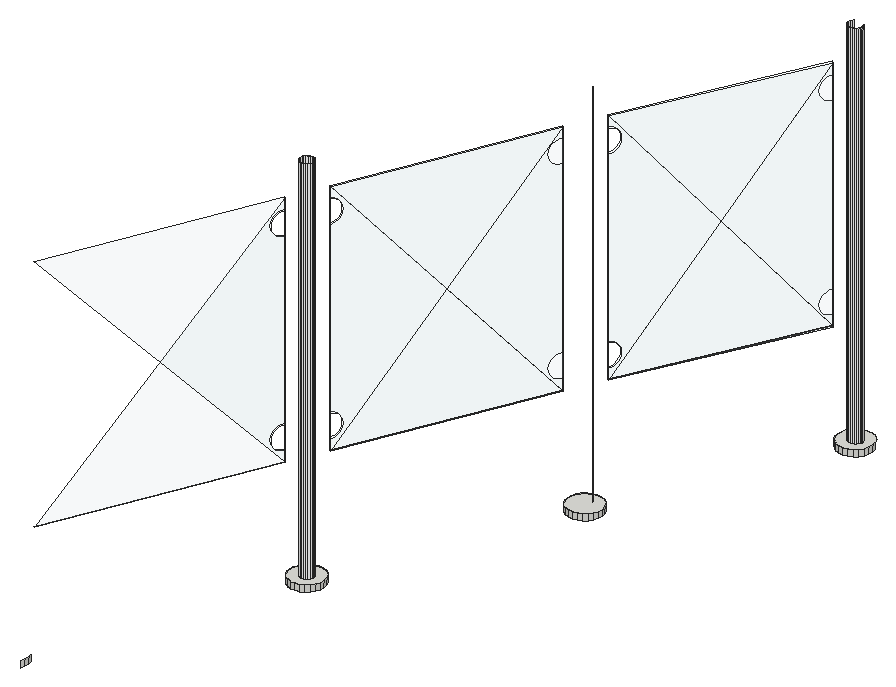
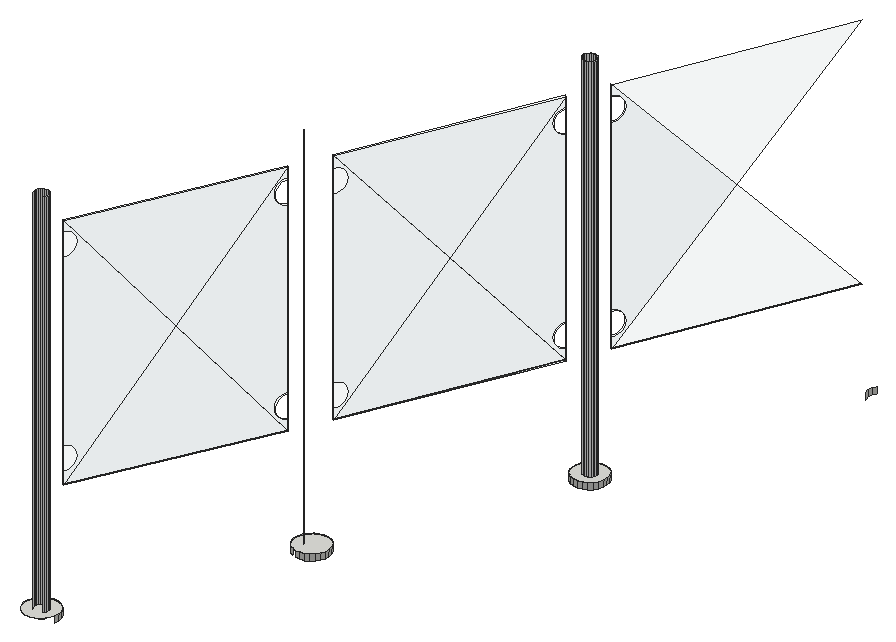
# SketchUp Ruby script. Lengths in inches.
U = 1.inch
M = Sketchup.active_model
def pt(a) = Geom::Point3d.new(a.map { |v| v * U })
def face(e, loops, mat)
  f = e.add_face(loops[0].map { |a| pt(a) })
  loops[1..].each { |l| e.add_face(l.map { |a| pt(a) }).erase! }
  f.material = f.back_material = mat if mat
  f
end
# faces: each face lists its corners as indices into pts; further lists are holes
def faces(e, pts, list, mat = nil) = list.each { |f| face(e, (f[0].is_a?(Array) ? f : [f]).map { |l| l.map { |i| pts[i] } }, mat) }
# xy, xz, yz: faces in a plane at the given z, y or x. An outline is a flat list of corners, or four numbers for a rectangle; further outlines are holes
def ring(l) = l.size == 4 ? [[l[0], l[1]], [l[2], l[1]], [l[2], l[3]], [l[0], l[3]]] : l.each_slice(2).to_a
def flat(e, list, mat, &to3) = list.each { |f| face(e, (f[0].is_a?(Array) ? f : [f]).map { |l| ring(l).map { |u, v| to3.(u, v) } }, mat) }
def xy(e, z, list, mat = nil) = flat(e, list, mat) { |x, y| [x, y, z] }
def xz(e, y, list, mat = nil) = flat(e, list, mat) { |x, z| [x, y, z] }
def yz(e, x, list, mat = nil) = flat(e, list, mat) { |y, z| [x, y, z] }
def lines(e, pts, list) = list.each { |a, b| e.add_line(pt(pts[a]), pt(pts[b])) }
# prism: a flat outline (further loops are holes) pulled along v
def prism(e, loops, v, mat = nil)
  f = face(e, loops, mat); d = Geom::Vector3d.new(v.map { |x| x * U })
  f.pushpull(f.normal.samedirection?(d) ? d.length : -d.length)
end
def box(e, o, s, mat = nil) = prism(e, [[o, [o[0] + s[0], o[1], o[2]], [o[0] + s[0], o[1] + s[1], o[2]], [o[0], o[1] + s[1], o[2]]]], [0, 0, s[2]], mat)
def at(x, y, z, deg = 0) = Geom::Transformation.translation(pt([x, y, z])) * Geom::Transformation.rotation(ORIGIN, Z_AXIS, deg.degrees)
def axes(o, x, y, z) = Geom::Transformation.new([*x, 0, *y, 0, *z, 0, *pt(o).to_a, 1])
def part(name) = M.definitions.add(name)
# library, detail: a bought-in or finely detailed component or shape, given as its bounding box
def library(name, o, s) = part(name).tap { |d| box(d.entities, o, s) }
def detail(e, o, s) = box(e.add_group.entities, o, s)
def put(e, d, t, mat = nil) = e.add_instance(d, t).tap { |i| i.material = mat if mat }
def group(e, t, mat = nil) = e.add_group.tap { |g| g.transformation = t; g.material = mat if mat }.entities
root = M.entities
M.materials.add("Glass_Safety_01").color = [204, 235, 244]
M.materials["Glass_Safety_01"].alpha = 0.1
M.materials.add("[Color_000]").color = [255, 255, 255]
xy(root,321.27,[[[936.05,747.22,936.45,747.3,936.82,747.48,937.13,747.75,937.36,748.1,937.48,748.49,937.51,748.9,937.43,749.3,937.24,749.67,936.97,749.98,936.625,750.2,936.5625,750.22,936.24,750.33,935.83,750.36,935.42,750.27,935.06,750.09,934.75,749.82,934.52,749.47,934.39,749.08,934.37,748.67,934.45,748.27,934.63,747.9,934.91,747.6,935.25,747.37,935.3125,747.35,935.64,747.24],[935.98,748.16,935.82,748.17,935.6875,748.21,935.66,748.22,935.53,748.31,935.42,748.43,935.34,748.58,935.31,748.74,935.32,748.91,935.37,749.0625,935.46,749.2,935.59,749.31,935.73,749.38,935.89,749.41,936.06,749.4,936.1875,749.36,936.21,749.35,936.35,749.26,936.46,749.14,936.53,748.99,936.57,748.83,936.56,748.67,936.51,748.51,936.41,748.375,936.29,748.26,936.14,748.19]],[935.3125,747.35,935.6875,748.21,935.66,748.22,935.53,748.31,935.42,748.43,935.34,748.58,935.31,748.74,935.32,748.91,935.37,749.0625,935.46,749.2,935.59,749.31,935.73,749.38,935.89,749.41,936.06,749.4,936.1875,749.36,936.5625,750.22,936.24,750.33,935.83,750.36,935.42,750.27,935.06,750.09,934.75,749.82,934.52,749.47,934.39,749.08,934.37,748.67,934.45,748.27,934.63,747.9,934.91,747.6,935.25,747.37],[935.6875,748.21,936.1875,749.36,936.06,749.4,935.89,749.41,935.73,749.38,935.59,749.31,935.46,749.2,935.37,749.0625,935.32,748.91,935.31,748.74,935.34,748.58,935.42,748.43,935.53,748.31,935.66,748.22]])
xy(root,321.27,[[935.98,748.16,936.14,748.19,936.29,748.26,936.41,748.375,936.51,748.51,936.56,748.67,936.57,748.83,936.53,748.99,936.46,749.14,936.35,749.26,936.21,749.35,936.1875,749.36,935.6875,748.21,935.82,748.17],[954.83,789.7,954.99,789.7,955.15,789.73,955.3,789.8,955.42,789.91,955.52,790.05,955.57,790.2,955.58,790.37,955.54,790.53,955.47,790.68,955.36,790.8,955.22,790.89,955.07,790.94,954.9,790.95,954.74,790.92,954.6,790.84,954.47,790.74,954.38,790.6,954.33,790.44,954.32,790.28,954.35,790.12,954.43,789.97,954.54,789.85,954.67,789.76]],"[Color_000]")
xy(root,321.86,[[936.05,747.22,936.45,747.3,936.82,747.48,937.13,747.75,937.36,748.1,937.48,748.49,937.51,748.9,937.43,749.3,937.24,749.67,936.97,749.98,936.625,750.2,936.24,750.33,935.83,750.36,935.42,750.27,935.06,750.09,934.75,749.82,934.52,749.47,934.39,749.08,934.37,748.67,934.45,748.27,934.63,747.9,934.91,747.6,935.25,747.37,935.64,747.24],[945.45,768.58,945.85,768.67,946.22,768.85,946.53,769.125,946.75,769.47,946.88,769.86,946.91,770.27,946.82,770.67,946.64,771.04,946.37,771.34,946.02,771.57,945.63,771.7,945.22,771.73,944.82,771.64,944.45,771.46,944.14,771.19,943.92,770.84,943.79,770.45,943.76,770.04,943.85,769.64,944.03,769.27,944.3,768.96,944.65,768.74,945.04,768.61],[955.0625,788.75,955.46,788.84,955.83,789.02,956.14,789.29,956.37,789.64,956.49,790.03,956.52,790.4375,956.4375,790.84,956.25,791.21,955.98,791.51,955.64,791.74,955.25,791.87,954.84,791.89,954.43,791.8125,954.07,791.63,953.76,791.35,953.53,791.01,953.4,790.62,953.38,790.21,953.46,789.81,953.64,789.44,953.92,789.13,954.26,788.91,954.65,788.78]])
xy(root,331.9,[[926.89,727.76,926.71,727.84,935.3,747.08],[926.71,727.84,935.125,747.16,935.3,747.08],[936.82,750.55,936.64,750.63,944.7,768.46],[936.64,750.63,944.52,768.54,944.7,768.46],[946.27,771.89,946.09,771.97,954.26,788.66],
  [946.09,771.97,954.09,788.75,954.26,788.66]],"Glass_Safety_01")
xz(root,789.7,[[954.83,321.27,954.99,357.27]],"[Color_000]")
p = [[927.43,725.31,321.27],[927.56,725.7,321.27],[927.56,725.7,321.86],[927.43,725.31,321.86],[927.58,726.11,321.27],[927.58,726.11,321.86],
  [927.5,726.51,321.27],[927.5,726.51,321.86],[935.25,747.37,321.27],[935.3125,747.35,321.27],[935.64,747.24,321.27],[935.64,747.24,321.86],
  [935.25,747.37,321.86],[936.05,747.22,321.27],[936.05,747.22,321.86],[936.45,747.3,321.27],[936.45,747.3,321.86],[936.82,747.48,321.27],
  [936.82,747.48,321.86],[934.91,747.6,321.27],[934.91,747.6,321.86],[937.13,747.75,321.27],[937.13,747.75,321.86],[934.63,747.9,321.27],
  [934.63,747.9,321.86],[937.36,748.1,321.27],[937.36,748.1,321.86],[934.45,748.27,321.27],[934.45,748.27,321.86],[937.48,748.49,321.27],
  [937.48,748.49,321.86],[935.53,748.31,321.27],[935.66,748.22,321.27],[935.66,748.22,357.27],[935.53,748.31,357.27],[935.6875,748.21,321.27],
  [935.82,748.17,321.27],[935.82,748.17,357.27],[935.98,748.16,321.27],[935.98,748.16,357.27],[936.14,748.19,321.27],[936.14,748.19,357.27],
  [936.29,748.26,321.27],[936.29,748.26,357.27],[934.37,748.67,321.27],[934.37,748.67,321.86],[935.42,748.43,321.27],[935.42,748.43,357.27],
  [936.41,748.375,321.27],[936.41,748.375,357.27],[935.34,748.58,321.27],[935.34,748.58,357.27],[936.51,748.51,321.27],[936.51,748.51,357.27],
  [936.56,748.67,321.27],[936.56,748.67,357.27],[937.51,748.9,321.27],[937.51,748.9,321.86],[935.31,748.74,321.27],[935.31,748.74,357.27],
  [934.39,749.08,321.27],[934.39,749.08,321.86],[935.32,748.91,321.27],[935.32,748.91,357.27],[936.57,748.83,321.27],[936.57,748.83,357.27],
  [936.53,748.99,321.27],[936.53,748.99,357.27],[935.37,749.0625,321.27],[935.37,749.0625,357.27],[937.43,749.3,321.27],[937.43,749.3,321.86],
  [936.46,749.14,321.27],[936.46,749.14,357.27],[934.52,749.47,321.27],[934.52,749.47,321.86],[935.46,749.2,321.27],[935.46,749.2,357.27],
  [936.35,749.26,321.27],[936.35,749.26,357.27],[935.59,749.31,321.27],[935.59,749.31,357.27],[935.73,749.38,321.27],[935.73,749.38,357.27],
  [936.21,749.35,321.27],[936.21,749.35,357.27],[937.24,749.67,321.27],[937.24,749.67,321.86],[935.89,749.41,321.27],[935.89,749.41,357.27],
  [936.06,749.4,321.27],[936.06,749.4,357.27],[936.1875,749.36,321.27],[934.75,749.82,321.27],[934.75,749.82,321.86],[936.97,749.98,321.27],
  [936.97,749.98,321.86],[935.06,750.09,321.27],[935.06,750.09,321.86],[936.625,750.2,321.27],[936.625,750.2,321.86],[935.42,750.27,321.27],
  [935.42,750.27,321.86],[936.5625,750.22,321.27],[936.24,750.33,321.27],[936.24,750.33,321.86],[935.83,750.36,321.27],[935.83,750.36,321.86],
  [944.65,768.74,321.27],[945.04,768.61,321.27],[945.04,768.61,321.86],[944.65,768.74,321.86],[945.45,768.58,321.27],[945.45,768.58,321.86],
  [945.85,768.67,321.27],[945.85,768.67,321.86],[944.3,768.96,321.27],[944.63,768.75,321.27],[944.3,768.96,321.86],[946.22,768.85,321.27],
  [946.22,768.85,321.86],[946.53,769.125,321.27],[946.53,769.125,321.86],[944.03,769.27,321.27],[944.03,769.27,321.86],[946.75,769.47,321.27],
  [946.75,769.47,321.86],[943.85,769.64,321.27],[943.85,769.64,321.86],[946.88,769.86,321.27],[946.88,769.86,321.86],[943.76,770.04,321.27],
  [943.76,770.04,321.86],[946.91,770.27,321.27],[946.91,770.27,321.86],[943.79,770.45,321.27],[943.79,770.45,321.86],[946.82,770.67,321.27],
  [946.82,770.67,321.86],[943.92,770.84,321.27],[943.92,770.84,321.86],[945.75,770.63,321.27],[945.61,770.72,321.27],[945.61,770.72,357.27],
  [945.75,770.63,357.27],[946.64,771.04,321.27],[946.64,771.04,321.86],[944.14,771.19,321.27],[944.14,771.19,321.86],[946.37,771.34,321.27],
  [946.37,771.34,321.86],[944.45,771.46,321.27],[944.45,771.46,321.86],[946.02,771.57,321.27],[946.02,771.57,321.86],[944.82,771.64,321.27],
  [944.82,771.64,321.86],[945.22,771.73,321.27],[945.22,771.73,321.86],[945.63,771.7,321.27],[945.63,771.7,321.86],[954.26,788.91,321.27],
  [954.65,788.78,321.27],[954.65,788.78,321.86],[954.26,788.91,321.86],[955.0625,788.75,321.27],[955.0625,788.75,321.86],[955.46,788.84,321.27],
  [955.46,788.84,321.86],[955.83,789.02,321.27],[955.83,789.02,321.86],[953.92,789.13,321.27],[953.92,789.13,321.86],[956.14,789.29,321.27],
  [956.14,789.29,321.86],[953.64,789.44,321.27],[953.64,789.44,321.86],[956.37,789.64,321.27],[956.37,789.64,321.86],[953.46,789.81,321.27],
  [953.46,789.81,321.86],[956.49,790.03,321.27],[956.49,790.03,321.86],[954.67,789.76,321.27],[954.83,789.7,321.27],[954.83,789.7,357.27],
  [954.67,789.76,357.27],[954.99,789.7,321.27],[955.15,789.73,321.27],[955.15,789.73,357.27],[954.99,789.7,357.27],[955.3,789.8,321.27],
  [955.3,789.8,357.27],[953.38,790.21,321.27],[953.38,790.21,321.86],[954.43,789.97,321.27],[954.54,789.85,321.27],[954.54,789.85,357.27],
  [954.43,789.97,357.27],[955.42,789.91,321.27],[955.42,789.91,357.27],[955.52,790.05,321.27],[955.52,790.05,357.27],[954.35,790.12,321.27],
  [954.35,790.12,357.27],[955.57,790.2,321.27],[955.57,790.2,357.27],[956.52,790.4375,321.27],[956.52,790.4375,321.86],[954.32,790.28,321.27],
  [954.32,790.28,357.27],[953.4,790.62,321.27],[953.4,790.62,321.86],[955.58,790.37,321.27],[955.58,790.37,357.27],[954.33,790.44,321.27],
  [954.33,790.44,357.27],[954.38,790.6,321.27],[954.38,790.6,357.27],[955.54,790.53,321.27],[955.54,790.53,357.27],[956.4375,790.84,321.27],
  [956.4375,790.84,321.86],[955.47,790.68,321.27],[955.47,790.68,357.27],[954.47,790.74,321.27],[954.47,790.74,357.27],[935.125,747.16,351.28],
  [935.125,747.16,335.125],[935.0625,747.02,335.125],[934.95,746.77,335.09],[934.85,746.53,334.98],[934.76,746.33,334.8125],[934.69,746.18,334.59],
  [934.65,746.08,334.34],[934.64,746.05,334.0625],[934.65,746.08,333.79],[934.69,746.18,333.53],[934.76,746.33,333.3125],[934.85,746.53,333.14],
  [934.95,746.77,333.04],[935.0625,747.02,333],[935.125,747.16,333],[935.125,747.16,331.9],[926.71,727.84,354.51],[935.125,747.16,354.51],
  [935.125,747.16,353.41],[935.0625,747.02,353.41],[934.95,746.77,353.37],[934.85,746.53,353.27],[934.76,746.33,353.1],[934.69,746.18,352.88],
  [934.65,746.08,352.62],[934.64,746.05,352.35],[934.65,746.08,352.07],[934.69,746.18,351.8125],[934.76,746.33,351.59],[934.85,746.53,351.43],
  [934.95,746.77,351.32],[935.0625,747.02,351.28],[935.3,747.08,331.9],[935.3,747.08,333],[935.24,746.94,333],[935.13,746.69,333.04],
  [935.03,746.45,333.14],[934.94,746.25,333.3125],[934.875,746.1,333.53],[934.83,746,333.79],[934.82,745.97,334.0625],[934.83,746,334.34],
  [934.875,746.1,334.59],[934.94,746.25,334.8125],[935.03,746.45,334.98],[935.13,746.69,335.09],[935.24,746.94,335.125],[935.3,747.08,335.125],
  [935.3,747.08,351.28],[935.24,746.94,351.28],[935.13,746.69,351.32],[935.03,746.45,351.43],[934.94,746.25,351.59],[934.875,746.1,351.8125],
  [934.83,746,352.07],[934.82,745.97,352.35],[934.83,746,352.62],[934.875,746.1,352.88],[934.94,746.25,353.1],[935.03,746.45,353.27],
  [935.13,746.69,353.37],[935.24,746.94,353.41],[935.3,747.08,353.41],[935.3,747.08,354.51],[926.89,727.76,331.9],[936.64,750.63,331.9],
  [936.82,750.55,331.9],[936.82,750.55,333],[936.82,750.55,335.125],[936.82,750.55,351.28],[936.82,750.55,353.41],[936.82,750.55,354.51],
  [936.64,750.63,354.51],[936.64,750.63,353.41],[936.64,750.63,351.28],[936.64,750.63,335.125],[936.64,750.63,333],[936.93,750.8,335.09],
  [937.03,751.03,334.98],[937.125,751.24,334.8125],[937.19,751.39,334.59],[937.23,751.49,334.34],[937.25,751.52,334.0625],[937.23,751.49,333.79],
  [937.19,751.39,333.53],[937.125,751.24,333.3125],[937.03,751.03,333.14],[936.93,750.8,333.04],[944.7,768.46,354.51],[936.93,750.8,353.37],
  [937.03,751.03,353.27],[937.125,751.24,353.1],[937.19,751.39,352.88],[937.23,751.49,352.62],[937.25,751.52,352.35],[937.23,751.49,352.07],
  [937.19,751.39,351.8125],[937.125,751.24,351.59],[937.03,751.03,351.43],[936.93,750.8,351.32],[944.7,768.46,331.9],[944.7,768.46,333],
  [944.7,768.46,335.125],[944.7,768.46,351.28],[944.7,768.46,353.41],[936.75,750.88,333.04],[936.85,751.11,333.14],[936.94,751.32,333.3125],
  [937.01,751.47,333.53],[937.05,751.57,333.79],[937.07,751.6,334.0625],[937.05,751.57,334.34],[937.01,751.47,334.59],[936.94,751.32,334.8125],
  [936.85,751.11,334.98],[936.75,750.88,335.09],[936.75,750.88,351.32],[936.85,751.11,351.43],[936.94,751.32,351.59],[937.01,751.47,351.8125],
  [937.05,751.57,352.07],[937.07,751.6,352.35],[937.05,751.57,352.62],[937.01,751.47,352.88],[936.94,751.32,353.1],[936.85,751.11,353.27],
  [936.75,750.88,353.37],[944.52,768.54,331.9],[944.52,768.54,351.28],[944.52,768.54,335.125],[944.45,768.39,335.125],[944.34,768.14,335.09],
  [944.24,767.91,334.98],[944.15,767.7,334.8125],[944.08,767.55,334.59],[944.04,767.45,334.34],[944.02,767.42,334.0625],[944.04,767.45,333.79],
  [944.08,767.55,333.53],[944.15,767.7,333.3125],[944.24,767.91,333.14],[944.34,768.14,333.04],[944.45,768.39,333],[944.52,768.54,333],
  [944.52,768.54,354.51],[944.52,768.54,353.41],[944.45,768.39,353.41],[944.34,768.14,353.37],[944.24,767.91,353.27],[944.15,767.7,353.1],
  [944.08,767.55,352.88],[944.04,767.45,352.62],[944.02,767.42,352.35],[944.04,767.45,352.07],[944.08,767.55,351.8125],[944.15,767.7,351.59],
  [944.24,767.91,351.43],[944.34,768.14,351.32],[944.45,768.39,351.28],[946.09,771.97,331.9],[946.27,771.89,331.9],[946.27,771.89,333],
  [946.27,771.89,335.125],[946.27,771.89,351.28],[946.27,771.89,353.41],[946.27,771.89,354.51],[946.09,771.97,354.51],[946.09,771.97,353.41],
  [946.09,771.97,351.28],[946.09,771.97,335.125],[946.09,771.97,333],[946.39,772.14,335.09],[946.5,772.37,334.98],[946.59,772.57,334.8125],
  [946.67,772.72,334.59],[946.71,772.82,334.34],[946.73,772.85,334.0625],[946.71,772.82,333.79],[946.67,772.72,333.53],[946.59,772.57,333.3125],
  [946.5,772.37,333.14],[946.39,772.14,333.04],[954.26,788.66,354.51],[946.39,772.14,353.37],[946.5,772.37,353.27],[946.59,772.57,353.1],
  [946.67,772.72,352.88],[946.71,772.82,352.62],[946.73,772.85,352.35],[946.71,772.82,352.07],[946.67,772.72,351.8125],[946.59,772.57,351.59],
  [946.5,772.37,351.43],[946.39,772.14,351.32],[954.26,788.66,331.9],[954.26,788.66,333],[954.19,788.5,333],[954.07,788.26,333.04],
  [953.96,788.02,333.14],[953.87,787.83,333.3125],[953.79,787.67,333.53],[953.75,787.58,333.79],[953.73,787.54,334.0625],[953.75,787.58,334.34],
  [953.79,787.67,334.59],[953.87,787.83,334.8125],[953.96,788.02,334.98],[954.07,788.26,335.09],[954.19,788.5,335.125],[954.26,788.66,335.125],
  [954.26,788.66,351.28],[954.19,788.5,351.28],[954.07,788.26,351.32],[953.96,788.02,351.43],[953.87,787.83,351.59],[953.79,787.67,351.8125],
  [953.75,787.58,352.07],[953.73,787.54,352.35],[953.75,787.58,352.62],[953.79,787.67,352.88],[953.87,787.83,353.1],[953.96,788.02,353.27],
  [954.07,788.26,353.37],[954.19,788.5,353.41],[954.26,788.66,353.41],[946.21,772.22,333.04],[946.32,772.45,333.14],[946.42,772.65,333.3125],
  [946.49,772.8,333.53],[946.53,772.9,333.79],[946.55,772.93,334.0625],[946.53,772.9,334.34],[946.49,772.8,334.59],[946.42,772.65,334.8125],
  [946.32,772.45,334.98],[946.21,772.22,335.09],[946.21,772.22,351.32],[946.32,772.45,351.43],[946.42,772.65,351.59],[946.49,772.8,351.8125],
  [946.53,772.9,352.07],[946.55,772.93,352.35],[946.53,772.9,352.62],[946.49,772.8,352.88],[946.42,772.65,353.1],[946.32,772.45,353.27],
  [946.21,772.22,353.37],[954.09,788.75,331.9],[954.09,788.75,354.51],[954.09,788.75,353.41],[954.09,788.75,351.28],[954.09,788.75,335.125],
  [954.09,788.75,333]]
faces(root,p,[[0,1,2,3],[1,4,5,2],[4,6,7,5],[8,9,10,11,12],[10,13,14,11],[13,15,16,14],[15,17,18,16],[19,8,12,20],
  [17,21,22,18],[23,19,20,24],[21,25,26,22],[27,23,24,28],[25,29,30,26],[44,27,28,45],[29,56,57,30],[60,44,45,61],
  [56,70,71,57],[74,60,61,75],[70,86,87,71],[93,74,75,94],[86,95,96,87],[97,93,94,98],[95,99,100,96],[101,97,98,102],
  [99,103,104,105,100],[106,101,102,107],[104,106,107,105],[108,109,110,111],[109,112,113,110],[112,114,115,113],[116,117,108,111,118],[114,119,120,115],
  [119,121,122,120],[123,116,118,124],[121,125,126,122],[127,123,124,128],[125,129,130,126],[131,127,128,132],[129,133,134,130],[135,131,132,136],
  [133,137,138,134],[139,135,136,140],[137,145,146,138],[147,139,140,148],[145,149,150,146],[151,147,148,152],[149,153,154,150],[155,151,152,156],
  [157,155,156,158],[159,157,158,160],[161,162,163,164],[162,165,166,163],[165,167,168,166],[167,169,170,168],[171,161,164,172],[169,173,174,170],
  [175,171,172,176],[173,177,178,174],[179,175,176,180],[177,181,182,178],[193,179,180,194],[181,207,208,182],[211,193,194,212],[207,221,222,208]])
faces(root,p,[[31,32,33,34],[32,35,36,37,33],[36,38,39,37],[38,40,41,39],[40,42,43,41],[46,31,34,47],[42,48,49,43],[50,46,47,51],
  [48,52,53,49],[52,54,55,53],[58,50,51,59],[62,58,59,63],[54,64,65,55],[64,66,67,65],[68,62,63,69],[66,72,73,67],
  [76,68,69,77],[72,78,79,73],[80,76,77,81],[82,80,81,83],[78,84,85,79],[88,82,83,89],[90,88,89,91],[84,92,90,91,85],
  [141,142,143,144],[183,184,185,186],[187,188,189,190],[188,191,192,189],[195,196,197,198],[196,183,186,197],[191,199,200,192],[199,201,202,200],
  [203,195,198,204],[201,205,206,202],[209,203,204,210],[205,213,214,206],[215,209,210,216],[217,215,216,218],[213,219,220,214],[219,223,224,220],
  [225,217,218,226]],"[Color_000]")
faces(root,p,[[227,228,229,230,231,232,233,234,235,236,237,238,239,240,241,242,243,244,245,246,247,248,249,250,251,252,253,254,255,256,257,258,259],[260,261,262,263,264,265,266,267,268,269,270,271,272,273,274,275,276,277,278,279,280,281,282,283,284,285,286,287,288,289,290,291,292],[260,243,242,228,227,246,245,291,290,276,275,261],[293,294,295,296,297,298,299,300,301,302,303,304],[297,296,305,306,307,308,309,310,311,312,313,314,315,295,294,316,299,298,317,318,319,320,321,322,323,324,325,326,327],[316,294,328,329,330,331,332],[293,304,333,334,335,336,337,338,339,340,341,342,343,303,302,344,345,346,347,348,349,350,351,352,353,354,301,300,355],[356,357,358,359,360,361,362,363,364,365,366,367,368,369,370,371,355,300,372,373,374,375,376,377,378,379,380,381,382,383,384,385,386],
  [328,355,371,357,356,373,372,316,332,331,330,329],[387,388,389,390,391,392,393,394,395,396,397,398],[391,390,399,400,401,402,403,404,405,406,407,408,409,389,388,410,393,392,411,412,413,414,415,416,417,418,419,420,421],[422,423,424,425,426,427,428,429,430,431,432,433,434,435,436,437,438,439,440,441,442,443,444,445,446,447,448,449,450,451,452,410,388],[387,398,453,454,455,456,457,458,459,460,461,462,463,397,396,464,465,466,467,468,469,470,471,472,473,474,395,394,475],[475,394,476,477,478,479,480],[422,475,480,479,478,477,476,410,452,438,437,423]],"Glass_Safety_01")
